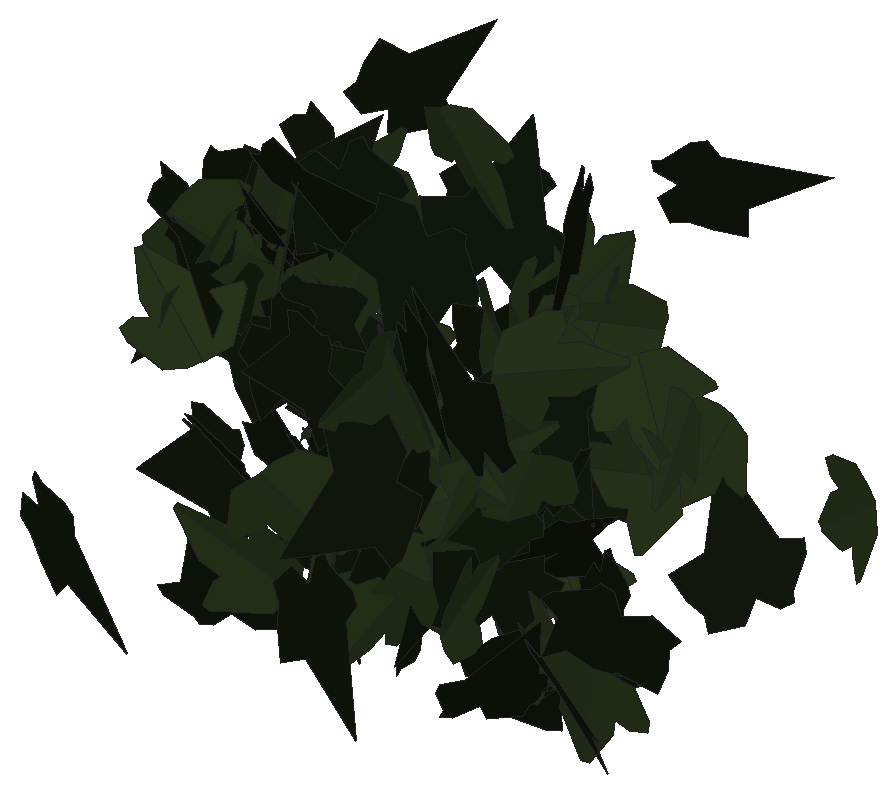
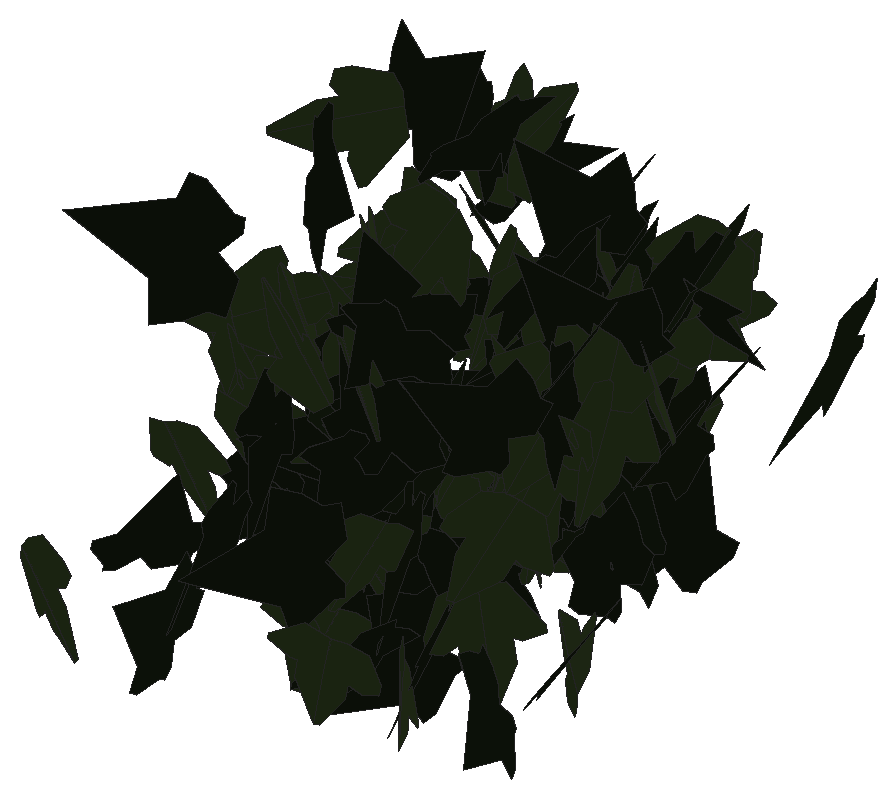
# SketchUp Ruby script. Lengths in inches.
U = 1.inch
M = Sketchup.active_model
def pt(a) = Geom::Point3d.new(a.map { |v| v * U })
def face(e, loops, mat)
  f = e.add_face(loops[0].map { |a| pt(a) })
  loops[1..].each { |l| e.add_face(l.map { |a| pt(a) }).erase! }
  f.material = f.back_material = mat if mat
  f
end
# faces: each face lists its corners as indices into pts; further lists are holes
def faces(e, pts, list, mat = nil) = list.each { |f| face(e, (f[0].is_a?(Array) ? f : [f]).map { |l| l.map { |i| pts[i] } }, mat) }
# xy, xz, yz: faces in a plane at the given z, y or x. An outline is a flat list of corners, or four numbers for a rectangle; further outlines are holes
def ring(l) = l.size == 4 ? [[l[0], l[1]], [l[2], l[1]], [l[2], l[3]], [l[0], l[3]]] : l.each_slice(2).to_a
def flat(e, list, mat, &to3) = list.each { |f| face(e, (f[0].is_a?(Array) ? f : [f]).map { |l| ring(l).map { |u, v| to3.(u, v) } }, mat) }
def xy(e, z, list, mat = nil) = flat(e, list, mat) { |x, y| [x, y, z] }
def xz(e, y, list, mat = nil) = flat(e, list, mat) { |x, z| [x, y, z] }
def yz(e, x, list, mat = nil) = flat(e, list, mat) { |y, z| [x, y, z] }
def lines(e, pts, list) = list.each { |a, b| e.add_line(pt(pts[a]), pt(pts[b])) }
# prism: a flat outline (further loops are holes) pulled along v
def prism(e, loops, v, mat = nil)
  f = face(e, loops, mat); d = Geom::Vector3d.new(v.map { |x| x * U })
  f.pushpull(f.normal.samedirection?(d) ? d.length : -d.length)
end
def box(e, o, s, mat = nil) = prism(e, [[o, [o[0] + s[0], o[1], o[2]], [o[0] + s[0], o[1] + s[1], o[2]], [o[0], o[1] + s[1], o[2]]]], [0, 0, s[2]], mat)
def at(x, y, z, deg = 0) = Geom::Transformation.translation(pt([x, y, z])) * Geom::Transformation.rotation(ORIGIN, Z_AXIS, deg.degrees)
def axes(o, x, y, z) = Geom::Transformation.new([*x, 0, *y, 0, *z, 0, *pt(o).to_a, 1])
def part(name) = M.definitions.add(name)
# library, detail: a bought-in or finely detailed component or shape, given as its bounding box
def library(name, o, s) = part(name).tap { |d| box(d.entities, o, s) }
def detail(e, o, s) = box(e.add_group.entities, o, s)
def put(e, d, t, mat = nil) = e.add_instance(d, t).tap { |i| i.material = mat if mat }
def group(e, t, mat = nil) = e.add_group.tap { |g| g.transformation = t; g.material = mat if mat }.entities
root = M.entities
M.materials.add("efeu1").color = [18, 25, 13]
M.materials.add("efeu2").color = [43, 57, 29]
c1 = part("ivyleaf_9")
p = [[1.54,2.16,1.25],[1.36,2.04,1.19],[-0.21,0.99,0.68],[-0.71,1.11,0.82],[-0.85,0.86,0.67],[-0.8,0.17,0.21],
  [-0.9,-0.01,0.1],[-0.67,-0.16,-0.02],[-0.08,-0.08,-0.05],[-0.03,-0.6,-0.4],[0.65,-0.88,-0.66],[0.83,-0.6,-0.49],
  [1.29,-0.42,-0.43],[1.8125,-0.07,-0.26],[1.21,0.44,0.15]]
faces(c1.entities,p,[[0,1,2,3,4,5,6,7,8,9,10,11,12,13,14]],"efeu1")
c2 = part("ivyleaf_10")
p = [[0,0.5,-0.03],[-0.0625,2.02,-0.43],[-0.19,2.01,-0.46],[-0.54,1.05,-0.29],[-0.52,0.625,-0.18],[-0.83,0.76,-0.28],
  [-1.16,0.64,-0.33],[-1.15,0.33,-0.24],[-0.77,-0.39,0.02],[-0.3,-0.51,0.16],[0.04,-0.48,0.23],[-0.02,2.01,-0.4375],
  [-0.06,2.01,-0.43],[0.04,-0.49,0.23],[0.67,-0.49,0.14],[1.38,0.36,-0.2],[1.375,0.51,-0.24],[0.81,0.65,-0.19],
  [0.62,0.59,-0.15],[0.6,1.09,-0.28],[0.5,1.23,-0.31]]
faces(c2.entities,p,[[0,1,2,3,4,5,6,7,8,9,10],[11,12,0,13,14,15,16,17,18,19,20]],"efeu2")
put(root,c1,axes([537.02,138.1,171.05],[-0.04755,-0.04459,0.76434],[0.6975,0.31328,0.06167],[-0.31573,0.6988,0.02112]))
put(root,c2,axes([537.43,134.6875,169.84],[-0.12711,-0.77879,-0.53764],[0.09255,0.52963,-0.78908],[0.94181,-0.15716,0.00498]))
put(root,c2,axes([537.15,133.73,169.5],[0.65861,-0.52729,-0.20055],[0.16142,-0.11926,0.84365],[-0.54055,-0.67806,0.00757]))
put(root,c1,axes([537.42,132.59,171.85],[0.2527,-0.34185,-0.84202],[-0.50154,0.67635,-0.42511],[0.75783,0.5616,-0.00057]))
put(root,c2,axes([537.7,134.5,170.34],[-0.40509,-0.76264,-0.38046],[-0.16341,-0.34393,0.86341],[-0.83646,0.43653,0.01558]))
put(root,c1,axes([537.56,136.1,170.85],[-0.35397,0.24305,-0.78912],[0.65672,-0.43755,-0.42935],[-0.5005,-0.74602,-0.00527]))
put(root,c1,axes([537.51,135.93,171.14],[-0.07013,-0.59841,0.53102],[0.00755,-0.53353,-0.60024],[0.80002,-0.04743,0.05221]))
put(root,c2,axes([537.5,131.98,171.7],[-0.39679,-0.49368,-0.65916],[0.44515,0.48701,-0.63271],[0.69286,-0.59562,0.02901]))
put(root,c1,axes([538.04,132.41,170.875],[-0.76463,-0.2128,0.03225],[-0.02822,-0.01885,-0.79362],[0.21337,-0.76508,0.01058]))
put(root,c1,axes([537.3125,132.64,171.34],[0.14558,-0.77645,0.53545],[0.20891,-0.50179,-0.78444],[0.91975,0.23688,0.09342]))
put(root,c2,axes([537.77,131.74,170.12],[0.07772,-0.8532,0.33575],[-0.04725,0.33278,0.85659],[-0.91567,-0.08959,-0.0157]))
put(root,c2,axes([538.27,131.14,170.11],[0.56501,0.55125,0.36674],[-0.27401,-0.24422,0.78923],[0.60274,-0.62777,0.01501]))
put(root,c2,axes([538.05,132.125,170.46],[-0.55578,-0.73185,-0.37562],[0.23045,0.29664,-0.91896],[0.78968,-0.60165,0.00382]))
put(root,c2,axes([538.15,135.88,170.79],[-0.03259,0.49166,0.71996],[-0.11998,0.71108,-0.49102],[-0.86352,-0.11735,0.04105]))
put(root,c2,axes([537.78,136.02,170.04],[0.67329,0.35045,0.38955],[0.34682,0.1774,-0.75903],[-0.39278,0.75736,-0.00246]))
put(root,c1,axes([537.84,134.29,170.67],[-0.38397,0.00007,0.79183],[0.79166,0.01836,0.38388],[-0.01649,0.87982,-0.00808]))
put(root,c1,axes([537.84,127.76,168.0625],[0.75304,-0.52934,-0.36142],[-0.28815,0.2185,-0.92039],[0.57253,0.8062,0.01214]))
put(root,c1,axes([538.46,136.49,164.69],[-0.00148,0.44784,0.67347],[-0.00202,0.67347,-0.44785],[-0.80878,-0.0025,-0.00012]))
put(root,c1,axes([538.32,133.74,170.29],[0.60748,-0.47511,0.2831],[-0.21819,0.18054,0.77117],[-0.50821,-0.64543,0.00731]))
put(root,c1,axes([537.99,133.47,168.95],[0.106,0.06134,0.80519],[0.74602,0.30343,-0.12133],[-0.30912,0.75333,-0.0167]))
put(root,c1,axes([537.96,133.76,170.3],[-0.01953,-0.14758,0.80337],[0.56749,-0.58043,-0.09283],[0.58748,0.55577,0.11638]))
put(root,c1,axes([537.93,133.97,166.18],[0.17836,-0.13445,0.78479],[0.60562,-0.4992,-0.22316],[0.5169,0.63127,-0.00933]))
put(root,c1,axes([538.2,134.68,165.07],[0.31453,-0.81616,-0.00549],[0.00961,0.00959,-0.87458],[0.81613,0.31443,0.01241]))
put(root,c2,axes([538.26,133.72,170.44],[0.45319,-0.30991,0.60783],[0.48871,-0.36174,-0.54881],[0.4761,0.66632,-0.01523]))
put(root,c1,axes([538.46,132.49,165.92],[-0.10256,0.82329,0.28892],[-0.01854,-0.2929,0.82805],[0.87232,0.09057,0.05157]))
put(root,c1,axes([538.18,131.62,167.98],[0.78369,-0.23894,0.08391],[0.08244,-0.01732,-0.81927],[0.23945,0.78798,0.00744]))
put(root,c1,axes([538.65,131.83,167.39],[0.32321,-0.71398,-0.4213],[0.16295,-0.38865,0.78366],[-0.81284,-0.36181,-0.01042]))
put(root,c2,axes([538.63,136.07,167.96],[-0.56269,-0.42029,-0.40052],[0.34496,0.2066,-0.70143],[0.46697,-0.65906,0.03554]))
put(root,c2,axes([538.35,134.47,164.37],[-0.26406,0.02088,0.74855],[0.66825,-0.35164,0.24554],[0.33795,0.71163,0.09937]))
put(root,c2,axes([538.54,133.46,171.6875],[0.52027,-0.48796,0.49163],[0.35005,-0.34535,-0.71322],[0.59771,0.62699,-0.01023]))
put(root,c2,axes([538.46,135.97,170.53],[0.60506,-0.22591,0.48774],[0.45371,-0.17913,-0.64581],[0.28822,0.75624,-0.00727]))
put(root,c2,axes([538.8,134.75,168.57],[-0.50407,-0.50077,-0.37122],[0.26274,0.26224,-0.71054],[0.56528,-0.56844,-0.00076]))
put(root,c2,axes([539.19,136.08,166.06],[-0.75867,-0.33026,0.21938],[-0.20089,-0.08816,-0.82743],[0.34182,-0.78481,0.00063]))
put(root,c1,axes([538.95,131.37,165.03],[0.67726,-0.00393,0.47864],[-0.47861,0.0059,0.67726],[-0.00661,-0.8293,0.00255]))
put(root,c2,axes([539.26,134.53,167.71],[-0.36175,-0.70482,-0.10935],[0.05407,0.09516,-0.79222],[0.7112,-0.36574,0.00461]))
put(root,c1,axes([538.67,134.14,167.9],[0.14576,-0.22383,0.84752],[0.45358,-0.71593,-0.26709],[0.7501,0.47642,-0.00318]))
put(root,c2,axes([539.17,132.77,165.68],[0.13622,-0.73977,-0.23015],[0.0391,-0.22682,0.7522],[-0.77376,-0.1417,-0.00251]))
put(root,c2,axes([539.57,137.57,165.43],[0.1333,-0.34067,-0.68513],[-0.24995,0.63791,-0.36582],[0.72318,0.28327,-0.00015]))
put(root,c1,axes([538.99,134.3,172.03],[0.30534,-0.83208,-0.39431],[-0.10527,0.38115,-0.88583],[0.91474,0.32161,0.02968]))
put(root,c1,axes([538.83,133.38,171.99],[0.09894,-0.31834,0.81653],[0.68942,-0.47905,-0.2703],[0.54107,0.6686,0.19511]))
put(root,c2,axes([539.25,135.28,169.32],[-0.17392,0.41093,-0.79478],[0.22499,-0.76355,-0.44402],[-0.86598,-0.28091,0.04426]))
put(root,c2,axes([540.26,130.6875,166.41],[-0.54796,-0.01997,-0.76744],[-0.76104,-0.1098,0.54625],[-0.10091,0.93657,0.04768]))
put(root,c1,axes([539.57,136.48,165.96],[0.44858,-0.41755,-0.51027],[-0.37682,0.34408,-0.61283],[0.54104,0.58583,-0.00375]))
put(root,c1,axes([539.18,132.46,170.11],[0.06163,-0.34853,-0.91107],[0.39475,0.84371,-0.29606],[0.89202,-0.34929,0.19396]))
put(root,c1,axes([539.17,133.39,166.98],[0.65029,-0.56004,0.19776],[0.14866,-0.13043,-0.85821],[0.57502,0.66707,-0.00177]))
put(root,c1,axes([539.6,133.48,169.49],[0.34575,-0.47064,-0.52274],[-0.31396,0.41797,-0.58398],[0.62944,0.467,-0.00415]))
put(root,c2,axes([540.03,133.46,170.84],[-0.67044,-0.47539,0.23155],[-0.18501,-0.13939,-0.82185],[0.49536,-0.69547,0.00644]))
put(root,c2,axes([539.51,139.62,166.6875],[0.75983,0.2131,0.24281],[0.23269,0.06947,-0.78914],[-0.2241,0.79465,0.00387]))
put(root,c1,axes([539.34,133.75,166.66],[0.09227,-0.06532,0.79458],[0.56614,-0.55783,-0.1116],[0.56135,0.57333,-0.01806]))
put(root,c1,axes([539.55,134.72,168.21],[0.30232,-0.90792,0.12651],[0.04317,-0.11897,-0.95693],[0.91568,0.30537,0.00335]))
put(root,c1,axes([540.04,131.15,170.77],[0.38633,-0.48176,-0.56583],[-0.32805,0.46166,-0.61705],[0.66681,0.50624,0.02425]))
put(root,c2,axes([539.92,132.71,165.8],[0.52239,-0.37085,0.59303],[0.48963,-0.33467,-0.6406],[0.49947,0.71594,0.00773]))
put(root,c2,axes([540.375,133.5,166.87],[0.49222,-0.71835,-0.05341],[-0.02405,0.04827,-0.87078],[0.71994,0.49276,0.00743]))
put(root,c1,axes([540.17,135.1875,166.34],[-0.5047,-0.43084,-0.58721],[0.49963,0.31499,-0.66054],[0.52991,-0.70734,0.06352]))
put(root,c2,axes([540.33,135.68,172.8],[-0.79227,0.23188,-0.40705],[0.39479,-0.10004,-0.82539],[-0.25219,-0.88508,-0.01335]))
put(root,c1,axes([540.6875,136.03,167.375],[0.51805,-0.08659,-0.63464],[-0.61169,0.17525,-0.52323],[0.19001,0.80027,0.04592]))
put(root,c1,axes([540.19,136.79,171.35],[-0.21381,-0.31415,-0.6767],[0.53125,0.43013,-0.36753],[0.52381,-0.56447,0.09654]))
put(root,c1,axes([540.17,136.14,165.05],[0.79102,0.05079,0.20048],[0.20013,0.01181,-0.79264],[-0.05213,0.81594,-0.00101]))
put(root,c1,axes([540.7,133.71,169.0625],[-0.30308,-0.7837,0.34392],[-0.12654,-0.3198,-0.84026],[0.84643,-0.32842,-0.00248]))
put(root,c1,axes([540.63,133.9375,164.09],[-0.19506,0.65819,0.57866],[0.14544,-0.56029,0.68632],[0.86424,0.24284,0.01511]))
put(root,c2,axes([540.66,136.99,167.34],[0.34576,0.59788,0.35399],[0.16398,0.31401,-0.69053],[-0.67519,0.38243,0.01357]))
put(root,c1,axes([540.71,137.66,165.45],[-0.13958,-0.76496,-0.11045],[0.03092,0.10662,-0.77751],[0.77228,-0.14253,0.01116]))
put(root,c2,axes([540.78,134.76,167.26],[-0.20707,0.37062,0.7211],[0.30487,-0.65404,0.4237],[0.75127,0.36757,0.02681]))
put(root,c1,axes([540.9,131.42,170.22],[0.30423,-0.64303,-0.3925],[0.19752,-0.34041,0.71078],[-0.727,-0.36158,0.02886]))
put(root,c1,axes([540.42,133.49,168.55],[0.04175,0.00111,-0.78786],[0.75539,0.2241,0.04035],[0.22384,-0.75647,0.01079]))
put(root,c1,axes([540.99,135.79,170.53],[-0.62839,-0.15266,0.58918],[0.59273,0.03886,0.64224],[-0.13825,0.86052,0.07552]))
put(root,c1,axes([540.99,135.53,167.55],[0.55264,-0.55946,0.01026],[-0.00721,0.00729,0.78638],[-0.5595,-0.55268,-0.00001]))
put(root,c2,axes([541.33,132.78,165.54],[-0.12309,-0.56005,0.66674],[-0.05284,-0.66732,-0.5703],[0.86914,-0.11989,0.05976]))
put(root,c2,axes([541.17,133.81,167.13],[0.05893,-0.24243,0.86025],[0.29745,-0.80766,-0.24798],[0.84281,0.30199,0.02737]))
put(root,c1,axes([540.77,138.34,167.44],[0.6183,0.06117,0.53264],[0.52419,0.10175,-0.62017],[-0.11258,0.80972,0.03769]))
put(root,c1,axes([541.24,134.74,166.01],[-0.01481,0.03185,-0.97254],[0.62332,-0.74658,-0.03394],[-0.7472,-0.62344,-0.00904]))
put(root,c1,axes([541.46,132.24,169.72],[-0.59598,-0.6159,-0.2281],[0.15687,0.16561,-0.85704],[0.63777,-0.61627,-0.00235]))
put(root,c1,axes([541.24,135.87,168.41],[-0.45265,-0.0354,0.74404],[0.6494,-0.44523,0.37389],[0.36487,0.74851,0.25759]))
put(root,c2,axes([541.72,136.33,170.34],[0.64143,-0.42974,-0.25223],[-0.19348,0.16409,-0.7716],[0.45919,0.66942,0.02721]))
put(root,c2,axes([541.42,129.52,169.07],[-0.56805,-0.47707,-0.52676],[0.43033,0.30578,-0.74099],[0.56559,-0.7118,0.03473]))
put(root,c2,axes([541.77,133.17,166.15],[-0.40734,-0.78012,-0.2349],[0.12234,0.20108,-0.87994],[0.80548,-0.42506,0.01486]))
put(root,c1,axes([541.6,135.79,167.99],[-0.22827,-0.41546,-0.67356],[0.30842,0.59889,-0.47393],[0.72882,-0.38357,-0.01041]))
put(root,c2,axes([542.18,131.42,169.58],[0.0991,-0.56246,-0.80506],[0.00773,0.80958,-0.56466],[0.98206,0.05038,0.08569]))
put(root,c1,axes([542.09,132.62,172.6],[-0.18992,-0.87616,0.1169],[-0.01244,-0.11691,-0.89642],[0.88383,-0.18991,0.0125]))
put(root,c2,axes([543.05,136.08,164.61],[0.10734,-0.03721,-0.82761],[-0.56836,0.60385,-0.10087],[0.60273,0.57604,0.05228]))
put(root,c2,axes([542.06,136.92,169.82],[0.64393,-0.29947,-0.58382],[0.52141,-0.26303,0.71002],[-0.39832,-0.82844,-0.01438]))
put(root,c2,axes([542.3,136.08,164.75],[0.62609,0.40959,0.3594],[0.3022,0.19454,-0.74816],[-0.45344,0.6952,-0.00239]))
put(root,c2,axes([542.02,131.66,167.75],[0.4327,-0.12005,-0.7589],[0.74542,-0.14557,0.44804],[-0.18628,-0.86138,0.03005]))
put(root,c1,axes([542.7,133.62,167.4],[-0.62517,-0.33633,0.57308],[0.58412,0.09693,0.69411],[-0.31677,0.84253,0.14891]))
put(root,c2,axes([542.05,134.34,170.15],[0.00957,-0.11853,0.97857],[0.9199,-0.35055,-0.05146],[0.35418,0.91368,0.10721]))
put(root,c2,axes([542.42,134.6875,170.64],[0.01394,-0.19207,-0.81099],[0.41304,-0.70289,0.17357],[-0.72387,-0.40477,0.08342]))
put(root,c2,axes([542.84,130.45,171.26],[-0.09068,-0.00456,-0.9556],[-0.0619,-0.95785,0.01044],[-0.95361,0.06261,0.0902]))
put(root,c1,axes([543.61,129.98,168.79],[-0.29518,0.58251,0.71709],[-0.39148,0.60302,-0.65099],[-0.83683,-0.48757,0.05159]))
put(root,c1,axes([542.5,129.07,167.65],[-0.26659,-0.15268,-0.86245],[0.8457,0.18967,-0.29499],[0.22787,-0.88256,0.08581]))
put(root,c1,axes([542.96,133.34,165.6],[-0.37831,-0.35315,0.72211],[0.62252,0.3762,0.51011],[-0.50855,0.72321,0.08726]))
put(root,c2,axes([543.56,133.88,165.03],[0.29308,-0.1675,-0.75225],[-0.59811,0.45809,-0.33503],[0.486,0.66477,0.04132]))
put(root,c1,axes([543.37,134.31,167.35],[-0.61127,0.51618,-0.29726],[-0.22788,0.19088,0.80006],[0.55034,0.65237,0.00111]))
put(root,c1,axes([542.82,134.45,169.28],[-0.04152,-0.64728,-0.63371],[0.06125,0.63092,-0.64845],[0.90378,-0.07249,0.01483]))
put(root,c1,axes([543.21,137.67,167.25],[0.24462,-0.08673,-0.76267],[-0.53436,0.55541,-0.23455],[0.55105,0.57709,0.11112]))
put(root,c2,axes([543.72,130.38,170.68],[-0.60492,0.37549,-0.48891],[-0.41069,0.26536,0.71195],[0.45973,0.73113,-0.00731]))
put(root,c2,axes([542.71,135.24,169.89],[0.00282,0.00453,-0.79912],[0.71087,-0.36508,0.00044],[-0.36507,-0.71085,-0.00532]))
put(root,c1,axes([543.87,132.8,168.23],[-0.57121,-0.14749,0.61094],[-0.58003,-0.19418,-0.58919],[0.242,-0.81353,0.02987]))
put(root,c2,axes([542.625,131.96,169.16],[-0.14415,-0.00685,-0.98136],[0.9105,-0.37106,-0.13115],[-0.3662,-0.91987,0.06021]))
put(root,c1,axes([543.27,134.05,166.48],[0.42145,0.65574,0.26194],[0.14451,0.21849,-0.77949],[-0.69117,0.44553,-0.00326]))
put(root,c2,axes([543.29,135.55,169.48],[0.34372,-0.75002,0.12988],[-0.05457,0.11786,0.82503],[-0.75923,-0.34803,-0.0005]))
put(root,c1,axes([543.625,135.78,167.65],[-0.68808,-0.47,0.07682],[-0.0585,-0.05055,-0.83323],[0.47263,-0.69051,0.00871]))
put(root,c2,axes([543.98,135.99,170.14],[-0.15793,-0.04586,-0.80992],[-0.69751,-0.4136,0.15943],[-0.41418,0.71403,0.04033]))
put(root,c1,axes([543.72,129.69,169.85],[-0.33706,-0.54818,0.64582],[-0.34393,-0.54665,-0.6435],[0.77414,-0.48154,-0.0047]))
put(root,c1,axes([543.22,132.78,164.14],[0.5853,0.57496,0.19386],[-0.14144,-0.13264,0.82045],[0.59005,-0.60213,0.00437]))
put(root,c1,axes([543.05,130.99,171.81],[0.00543,-0.03981,-0.82611],[0.82707,0.00006,0.00543],[-0.0002,-0.82613,0.03981]))
put(root,c1,axes([543.02,139.48,165.69],[0.39898,-0.53124,0.52752],[0.30741,-0.42879,-0.66432],[0.68264,0.50359,-0.00916]))
put(root,c1,axes([543.35,135.19,172.67],[-0.26487,0.10889,-0.94777],[0.81942,-0.47774,-0.28389],[-0.48854,-0.86034,0.03769]))
put(root,c1,axes([543.73,135.86,168.33],[0.59203,-0.06235,-0.60081],[-0.59929,0.0446,-0.59516],[0.07556,0.84231,-0.01296]))
put(root,c1,axes([543.07,133.48,164.08],[0.38092,-0.06687,0.7994],[0.80144,-0.00645,-0.38243],[0.03461,0.88549,0.05758]))
put(root,c2,axes([544.24,132.66,168.99],[-0.59307,-0.57129,0.255],[-0.18424,-0.1763,-0.82347],[0.59787,-0.62103,-0.00081]))
put(root,c2,axes([543.92,132.38,169.32],[0.12961,-0.45824,0.7792],[0.1809,-0.7581,-0.47592],[0.88567,0.2219,-0.01682]))
put(root,c2,axes([544.69,135.39,167.83],[0.26012,-0.05093,-0.9672],[-0.93863,0.23369,-0.26474],[0.23882,0.97392,0.01294]))
put(root,c2,axes([543.88,131.47,169.55],[0.13109,-0.20385,0.83717],[0.14266,0.84025,0.18226],[-0.84974,0.10962,0.15975]))
put(root,c1,axes([543.78,135.21,165.61],[-0.24112,-0.05773,-0.76486],[0.76477,0.04346,-0.24438],[0.05889,-0.80079,0.04187]))
put(root,c1,axes([543.63,137.63,172.04],[0.4362,0.45354,-0.61978],[0.36716,0.50289,0.62641],[0.67455,-0.56701,0.05982]))
put(root,c2,axes([544.54,130.41,167.16],[0.11601,-0.1999,0.80285],[-0.36489,0.71524,0.23081],[-0.74255,-0.3827,0.012]))
put(root,c2,axes([544.68,137.1875,167.86],[0.74624,-0.17636,-0.26112],[-0.25159,0.07067,-0.76673],[0.18972,0.78744,0.01033]))
put(root,c1,axes([545.07,130.4,170.77],[0.22847,-0.3124,0.89181],[-0.52664,0.71971,0.38703],[-0.78459,-0.57406,-0.00009]))
put(root,c2,axes([544.93,133.59,164.73],[-0.8563,-0.1523,0.23958],[-0.23601,-0.04125,-0.86974],[0.15779,-0.88823,-0.00069]))
put(root,c2,axes([544.45,135.47,169.55],[0.60603,0.53614,0.23703],[0.16982,0.16573,-0.80907],[-0.56106,0.62927,0.01114]))
put(root,c1,axes([545.16,133.94,165.88],[0.13554,0.30212,-0.80226],[-0.45139,-0.66536,-0.32683],[-0.72879,0.46829,0.05322]))
put(root,c1,axes([544.25,133.41,164.68],[0.32247,-0.57829,0.62565],[0.35595,-0.51634,-0.66071],[0.77405,0.47835,0.04319]))
put(root,c2,axes([545.25,135.46,169.05],[0.74873,-0.40509,-0.04828],[-0.04226,0.02335,-0.85129],[0.40576,0.74992,0.00043]))
put(root,c1,axes([545.63,136.95,165.27],[-0.58915,-0.49016,0.28574],[0.21901,0.18352,0.76639],[-0.52339,0.62854,-0.00095]))
put(root,c2,axes([544.91,131.62,171.62],[-0.1049,-0.05217,-0.90399],[0.70511,0.56623,-0.1145],[0.56809,-0.71244,-0.02481]))
put(root,c2,axes([545.96,139.36,165.95],[0.46537,-0.31699,-0.65978],[-0.50248,0.43017,-0.5611],[0.53227,0.68325,0.04716]))
